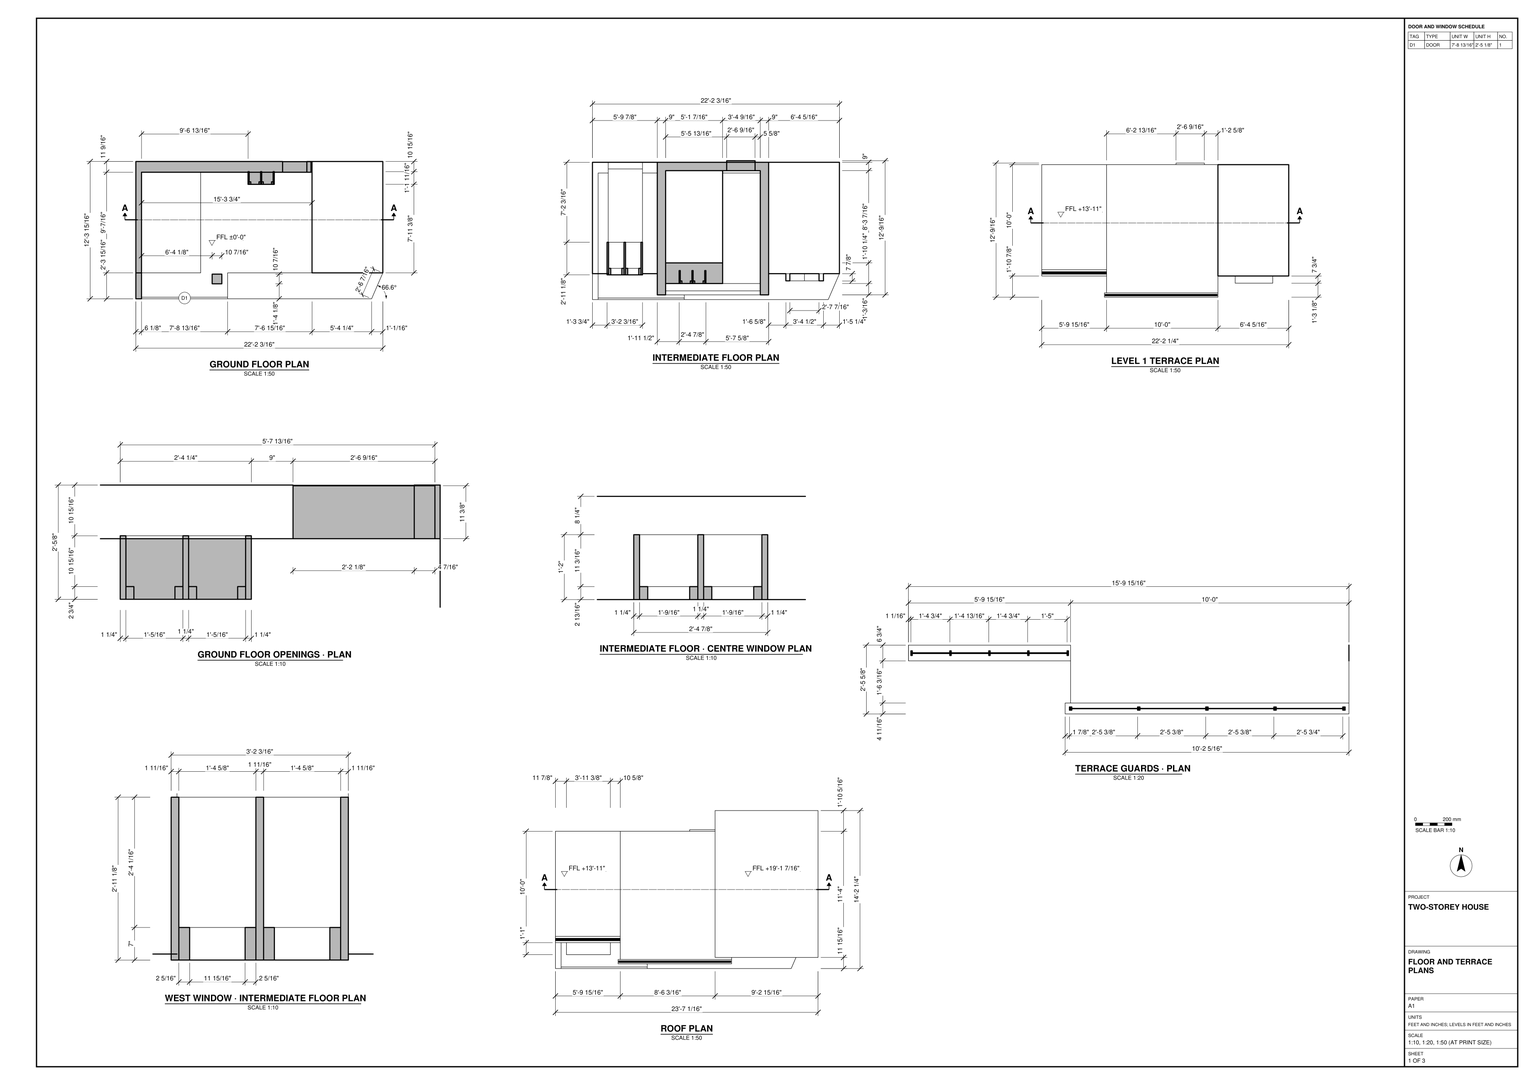
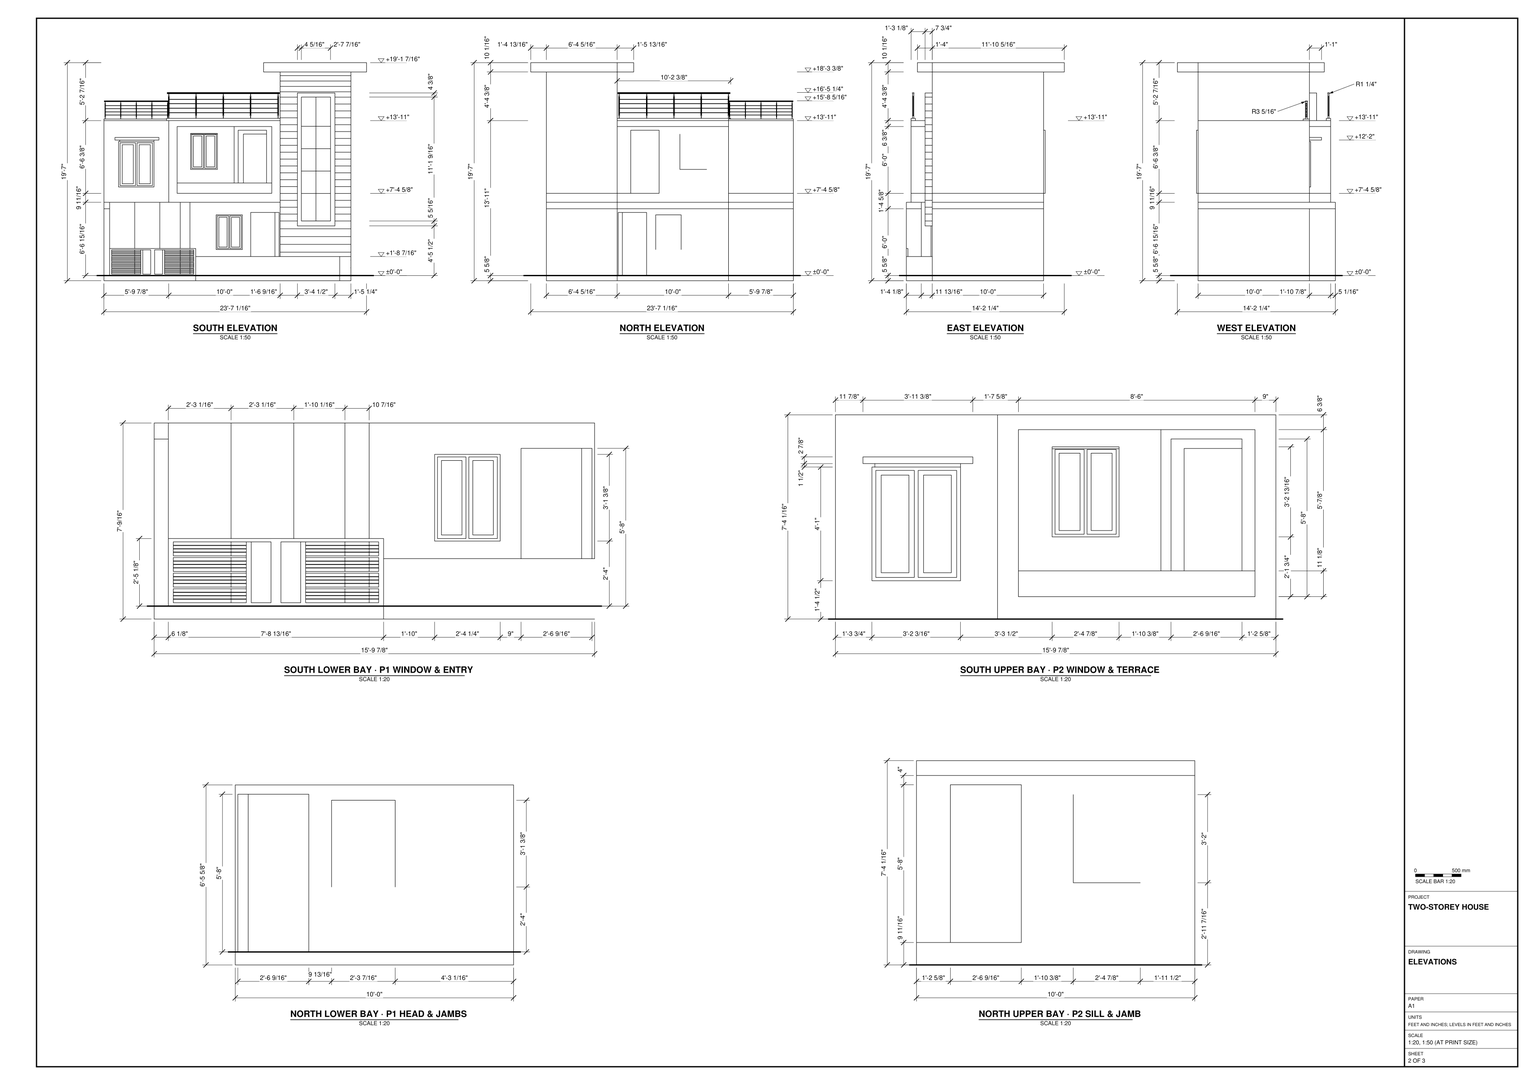
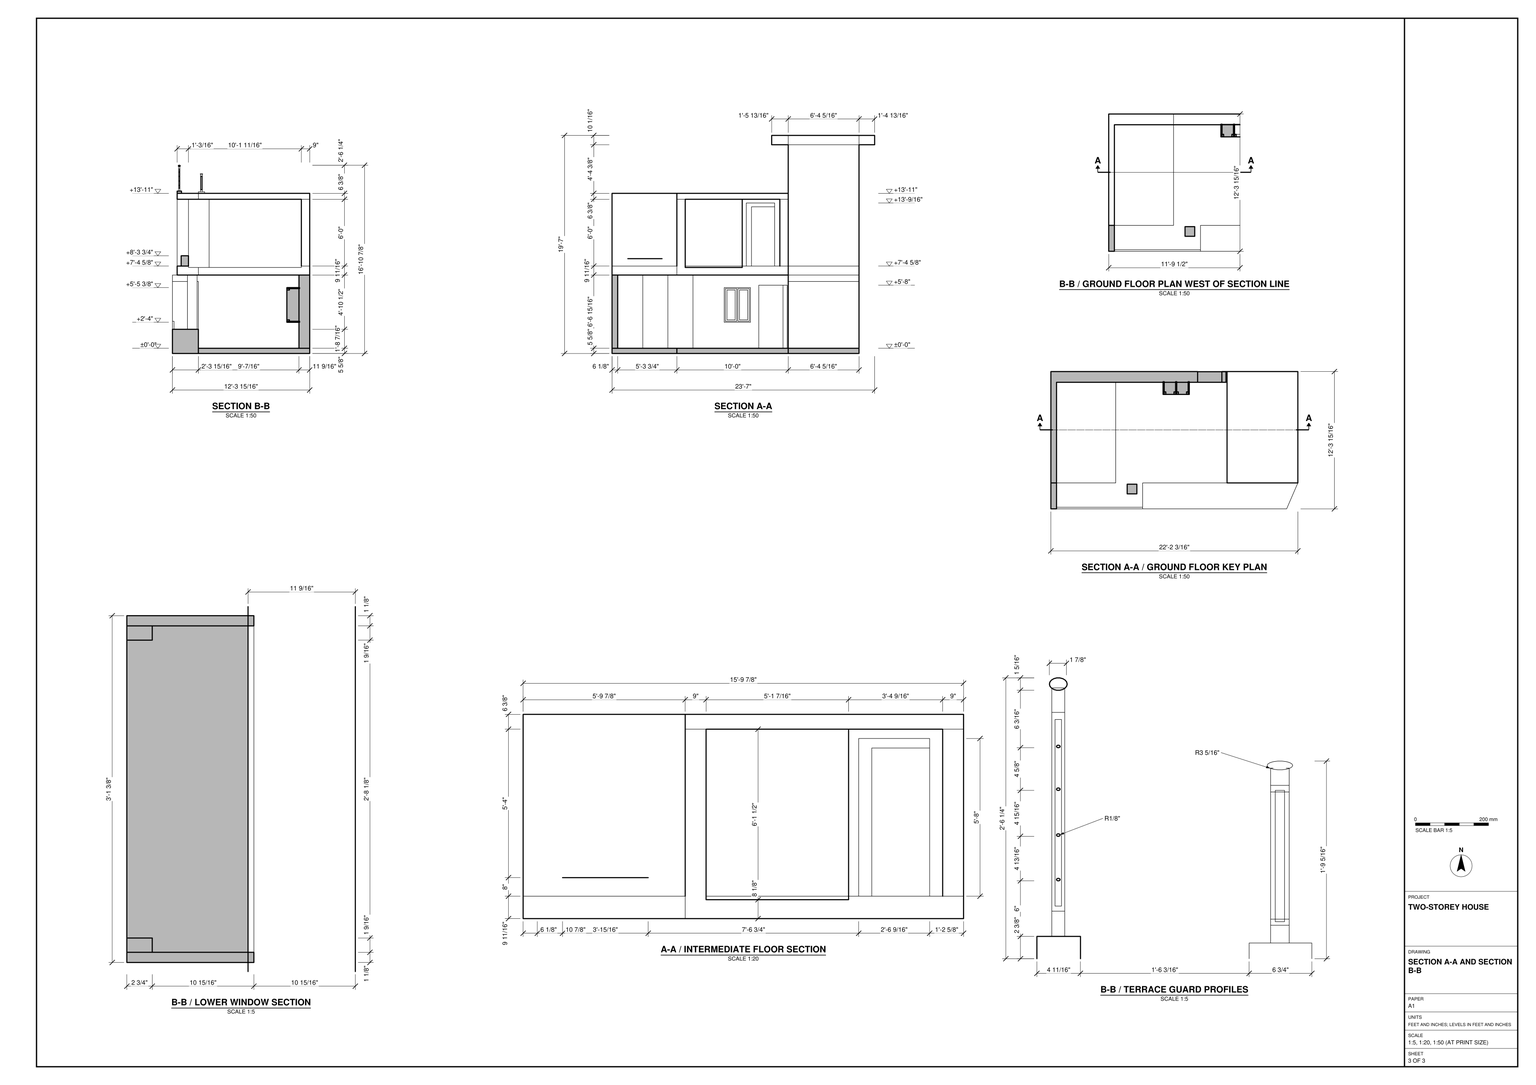
Build the two-storey house in SketchUp from task_files/diagram_01.pdf. Work in feet and inches. The overall size is 23'-7 1/16" east to west, 14'-2 1/4" north to south and 19'-7" high. Set the ground floor at ±0'-0" and the terrace at +13'-11". Use the sections to place the intermediate floor between these levels and to establish the slab thicknesses.

Follow the footprints on the floor plans, including the angled corner at the southeast of the ground floor. Give the walls their drawn thicknesses and form the door and window openings with their frames, sills and recesses. On the south elevation, model the low entry gate, the upper west window beneath its projecting head, and the recessed upper bay with a window and door. Give the taller east bay its horizontal bands, tall divided window and overhanging flat roof. Follow the terrace plan for the offset guard runs and the elevations for their different heights.

Keep the walls, slabs and roof as separate groups or components, and group each joinery or furniture piece separately where shown. Use components for repeated parts. Any decor or loose items may be suitable library components. Save one SketchUp model as output_files/two_storey_house_with_stepped_terraces_and_a_tower_bay.skp.

# SketchUp Ruby script. Lengths in inches.
U = 1.inch
M = Sketchup.active_model
def pt(a) = Geom::Point3d.new(a.map { |v| v * U })
def face(e, loops, mat)
  f = e.add_face(loops[0].map { |a| pt(a) })
  loops[1..].each { |l| e.add_face(l.map { |a| pt(a) }).erase! }
  f.material = f.back_material = mat if mat
  f
end
# faces: each face lists its corners as indices into pts; further lists are holes
def faces(e, pts, list, mat = nil) = list.each { |f| face(e, (f[0].is_a?(Array) ? f : [f]).map { |l| l.map { |i| pts[i] } }, mat) }
# xy, xz, yz: faces in a plane at the given z, y or x. An outline is a flat list of corners, or four numbers for a rectangle; further outlines are holes
def ring(l) = l.size == 4 ? [[l[0], l[1]], [l[2], l[1]], [l[2], l[3]], [l[0], l[3]]] : l.each_slice(2).to_a
def flat(e, list, mat, &to3) = list.each { |f| face(e, (f[0].is_a?(Array) ? f : [f]).map { |l| ring(l).map { |u, v| to3.(u, v) } }, mat) }
def xy(e, z, list, mat = nil) = flat(e, list, mat) { |x, y| [x, y, z] }
def xz(e, y, list, mat = nil) = flat(e, list, mat) { |x, z| [x, y, z] }
def yz(e, x, list, mat = nil) = flat(e, list, mat) { |y, z| [x, y, z] }
def lines(e, pts, list) = list.each { |a, b| e.add_line(pt(pts[a]), pt(pts[b])) }
# prism: a flat outline (further loops are holes) pulled along v
def prism(e, loops, v, mat = nil)
  f = face(e, loops, mat); d = Geom::Vector3d.new(v.map { |x| x * U })
  f.pushpull(f.normal.samedirection?(d) ? d.length : -d.length)
end
def box(e, o, s, mat = nil) = prism(e, [[o, [o[0] + s[0], o[1], o[2]], [o[0] + s[0], o[1] + s[1], o[2]], [o[0], o[1] + s[1], o[2]]]], [0, 0, s[2]], mat)
def at(x, y, z, deg = 0) = Geom::Transformation.translation(pt([x, y, z])) * Geom::Transformation.rotation(ORIGIN, Z_AXIS, deg.degrees)
def axes(o, x, y, z) = Geom::Transformation.new([*x, 0, *y, 0, *z, 0, *pt(o).to_a, 1])
def part(name) = M.definitions.add(name)
# library, detail: a bought-in or finely detailed component or shape, given as its bounding box
def library(name, o, s) = part(name).tap { |d| box(d.entities, o, s) }
def detail(e, o, s) = box(e.add_group.entities, o, s)
def put(e, d, t, mat = nil) = e.add_instance(d, t).tap { |i| i.material = mat if mat }
def group(e, t, mat = nil) = e.add_group.tap { |g| g.transformation = t; g.material = mat if mat }.entities
root = M.entities
M.materials.add("JJJ1").color = [238, 218, 183]
M.materials.add("MU TIGHI 6T67L 1").color = [235, 235, 235]
M.materials.add("T ER5Y 565N 1").color = [201, 111, 22]
M.materials.add("T R72 56 8, 7 5U1").color = [25, 25, 25]
M.materials.add("[Color I02]").color = [170, 141, 255]
M.materials["[Color I02]"].alpha = 0.92
M.materials.add("[Color J02]").color = [244, 207, 255]
M.materials.add("[Color J07]").color = [2, 0, 62]
M.materials.add("[Color M08]").color = [30, 30, 30]
M.materials.add("[Translucent Glass Blue]").color = [100, 149, 237]
M.materials["[Translucent Glass Blue]"].alpha = 0.18
M.materials.add("[Translucent Glass Gray]1").color = [132, 132, 132]
M.materials["[Translucent Glass Gray]1"].alpha = 0.25
M.materials.add("[Wood Plywood Knots]").color = [137, 122, 41]
M.materials.add("[Wood Veneer 01]").color = [120, 70, 37]
M.materials.add("wefsd tger 1").color = [92, 92, 92]
c1 = part("Group\#8")
xy(c1.entities,0,[[0,0,19.69,1.18]],"[Wood Veneer 01]")
xy(c1.entities,2.76,[[2.76,0,16.93,1.18]],"[Wood Veneer 01]")
xy(c1.entities,60.24,[[2.76,0,16.93,1.18]],"[Wood Veneer 01]")
xy(c1.entities,62.99,[[0,0,19.69,1.18]],"[Wood Veneer 01]")
xz(c1.entities,0,[[2.76,2.76,16.93,60.24]],"[Translucent Glass Gray]1")
xz(c1.entities,0,[[[0,0,19.69,62.99],[2.76,2.76,16.93,60.24]]],"[Wood Veneer 01]")
xz(c1.entities,1.18,[[[0,0,19.69,62.99],[2.76,2.76,16.93,60.24]]],"[Wood Veneer 01]")
yz(c1.entities,0,[[0,0,1.18,62.99]],"[Wood Veneer 01]")
yz(c1.entities,2.76,[[0,2.76,1.18,60.24]],"[Wood Veneer 01]")
yz(c1.entities,16.93,[[0,2.76,1.18,60.24]],"[Wood Veneer 01]")
yz(c1.entities,19.69,[[0,0,1.18,62.99]],"[Wood Veneer 01]")
c2 = part("pintu 2")
put(c2.entities,c1,at(-19.69,0,1.97))
g1 = group(c2.entities,at(-21.65,0,0))
prism(g1,[[[0,0,66.93],[0,0,0],[45.28,0,0],[45.28,0,66.93]],[[43.31,0,1.97],[23.62,0,1.97],[23.62,0,64.96],[43.31,0,64.96]],[[21.65,0,64.96],[21.65,0,1.97],[1.97,0,1.97],[1.97,0,64.96]]],[0,5.91,0],"[Wood Veneer 01]")
put(c2.entities,c1,at(1.97,0,1.97))
c3 = part("DOOR12")
g2 = group(c3.entities,at(114.73,28.14,-0.51))
g3 = group(g2,at(0,0,0))
box(g3,[0,0,0],[36,0.5,77.7])
c4 = part("Box01")
box(c4.entities,[-251.12,-5.93,-8.91],[582.61,12.27,8.91],"wefsd tger 1")
c5 = part("Box45")
box(c5.entities,[-240.91,-0.82,12.1],[2.44,1.82,74.48],"JJJ1")
c6 = part("Cylinder01")
prism(c6.entities,[[[328.21,-1.16,98.56],[328.21,-0.34,98.26],[328.21,0.53,98.26],[328.21,1.34,98.56],[328.21,2.01,99.11],[328.21,2.44,99.87],[328.21,2.59,100.72],[328.21,2.44,101.58],[328.21,2.01,102.33],[328.21,1.34,102.89],[328.21,0.53,103.18],[328.21,-0.34,103.18],[328.21,-1.16,102.89],[328.21,-1.82,102.33],[328.21,-2.25,101.58],[328.21,-2.41,100.72],[328.21,-2.25,99.87],[328.21,-1.82,99.11]]],[-576.3,0,0],"T ER5Y 565N 1")
c7 = part("Cylinder02")
prism(c7.entities,[[[-239.93,0.18,76.32],[-239.93,0.34,76.26],[-239.93,0.48,76.15],[-239.93,0.5625,75.99],[-239.93,0.59,75.82],[-239.93,0.5625,75.65],[-239.93,0.48,75.5],[-239.93,0.34,75.39],[-239.93,0.18,75.33],[-239.93,0.01,75.33],[-239.93,-0.16,75.39],[-239.93,-0.29,75.5],[-239.93,-0.375,75.65],[-239.93,-0.41,75.82],[-239.93,-0.375,75.99],[-239.93,-0.29,76.15],[-239.93,-0.16,76.26],[-239.93,0.01,76.32]]],[560.05,0,0],"T R72 56 8, 7 5U1")
c8 = part("Rectangle1")
prism(c8.entities,[[[-237.41,1.91,10.08],[-239.22,1.91,10.08],[-239.22,1.91,0.02],[-240.41,1.91,0.02],[-240.41,1.91,10.08],[-242.22,1.91,10.08],[-242.22,1.91,89.41],[-240.41,1.91,89.41],[-240.41,1.91,99.1875],[-239.22,1.91,99.1875],[-239.22,1.91,89.41],[-237.41,1.91,89.41]],[[-240.4375,1.91,85.68],[-240.4375,1.91,13.53],[-239.08,1.91,13.53],[-239.08,1.91,85.68]]],[0,-3.64,0],"MU TIGHI 6T67L 1")
c9 = part("skp243")
put(c9.entities,c4,at(0,0,0))
put(c9.entities,c5,at(0,0,0))
put(c9.entities,c6,at(0,0,0))
put(c9.entities,c7,at(0,0,0))
put(c9.entities,c8,at(0,0,0))
put(c9.entities,c7,at(0,0,-17.07))
put(c9.entities,c7,at(0,0,-35.38))
put(c9.entities,c7,at(0,0,-53.15))
put(c9.entities,c5,at(139.83,0,0))
put(c9.entities,c8,at(139.83,0,0))
put(c9.entities,c8,at(279.78,0,0))
put(c9.entities,c5,at(279.78,0,0))
put(c9.entities,c5,at(419.57,0,0))
put(c9.entities,c8,at(419.57,0,0))
put(c9.entities,c8,at(561.11,0,0))
put(c9.entities,c5,at(561.11,0,0))
c10 = part("Railing1")
put(c10.entities,c9,at(251.12,5.93,8.91))
c11 = part("1")
xy(c11.entities,0,[[0,0,58.27,0.39]])
xy(c11.entities,0.39,[[0,0,58.27,0.39]])
xy(c11.entities,3.9375,[[0,0,58.27,0.39]])
xy(c11.entities,4.33,[[0,0,58.27,0.39]])
xy(c11.entities,7.875,[[0,0,58.27,0.39]])
xy(c11.entities,8.27,[[0,0,58.27,0.39]])
xz(c11.entities,0,[[0,0,58.27,0.39],[0,3.9375,58.27,4.33],[0,7.875,58.27,8.27]])
xz(c11.entities,0.39,[[0,0,58.27,0.39],[0,3.9375,58.27,4.33],[0,7.875,58.27,8.27]])
c12 = part("gate")
xy(c12.entities,0,[[0,0,171.26,1.97]])
xy(c12.entities,3.9375,[[3.9375,0,62.01,1.97],[65.94,0,81.69,0.39],[89.57,0,105.31,0.39],[109.25,0,167.32,1.97],[65.94,0.98,81.69,1.97],
  [89.57,0.98,105.31,1.97]])
xy(c12.entities,20.18,[[3.9375,0,62.01,1.97],[109.25,0,167.32,1.97]])
xy(c12.entities,22.15,[[3.9375,0,62.01,1.97],[109.25,0,167.32,1.97]])
xy(c12.entities,38.39,[[3.9375,0,62.01,1.97],[109.25,0,167.32,1.97]])
xy(c12.entities,40.35,[[3.9375,0,62.01,1.97],[109.25,0,167.32,1.97]])
xy(c12.entities,56.59,[[3.9375,0,62.01,1.97],[109.25,0,167.32,1.97]])
xy(c12.entities,58.5625,[[3.9375,0,62.01,1.97],[109.25,0,167.32,1.97]])
xy(c12.entities,62.6,[[3.9375,0.59,62.2,0.98]])
xy(c12.entities,62.99,[[3.9375,0.59,62.2,0.98]])
xy(c12.entities,66.54,[[3.9375,0.59,62.2,0.98]])
xy(c12.entities,66.93,[[3.9375,0.59,62.2,0.98]])
xy(c12.entities,70.47,[[3.9375,0.59,62.2,0.98]])
xy(c12.entities,70.87,[[3.9375,0.59,62.2,0.98]])
xy(c12.entities,74.8,[[3.9375,0,62.01,1.97],[65.94,0,81.69,0.39],[89.57,0,105.31,0.39],[109.25,0,167.32,1.97],[65.94,0.98,81.69,1.97],
  [89.57,0.98,105.31,1.97]])
xy(c12.entities,78.74,[[0,0,171.26,1.97]])
xz(c12.entities,0,[[[0,0,85.63,78.74],[65.94,3.9375,81.69,74.8],[3.9375,22.15,62.01,38.39],[3.9375,3.9375,62.01,20.18],[3.9375,58.5625,62.01,74.8],[3.9375,40.35,62.01,56.59]],[[85.63,0,171.26,78.74],[89.57,3.9375,105.31,74.8],[109.25,22.15,167.32,38.39],[109.25,40.35,167.32,56.59],[109.25,58.5625,167.32,74.8],[109.25,3.9375,167.32,20.18]]],"[Color M08]")
xz(c12.entities,0.39,[[65.94,3.9375,81.69,74.8],[89.57,3.9375,105.31,74.8]],"[Wood Plywood Knots]")
xz(c12.entities,0.59,[[3.9375,62.6,62.2,62.99],[3.9375,66.54,62.2,66.93],[3.9375,70.47,62.2,70.87]])
xz(c12.entities,0.98,[[65.94,3.9375,81.69,74.8],[89.57,3.9375,105.31,74.8],[3.9375,62.6,62.2,62.99],[3.9375,66.54,62.2,66.93],[3.9375,70.47,62.2,70.87]])
xz(c12.entities,1.97,[[[0,0,171.26,78.74],[65.94,3.9375,81.69,74.8],[89.57,3.9375,105.31,74.8],[109.25,40.35,167.32,56.59],[109.25,22.15,167.32,38.39],[3.9375,3.9375,62.01,20.18],[3.9375,22.15,62.01,38.39],[109.25,58.5625,167.32,74.8],[3.9375,40.35,62.01,56.59],[3.9375,58.5625,62.01,74.8],[109.25,3.9375,167.32,20.18]]])
yz(c12.entities,0,[[0,0,1.97,78.74]])
yz(c12.entities,3.9375,[[0,3.9375,0.98,20.18],[0.98,3.9375,1.97,20.18],[0,22.15,0.98,38.39],[0.98,22.15,1.97,38.39],[0,40.35,0.98,56.59],
  [0.98,40.35,1.97,56.59],[0,58.5625,0.98,58.5625,0.98,62.6,0.59,62.6,0.59,62.99,0.98,62.99,0.98,66.54,0.59,66.54,0.59,66.93,0.98,66.93,0.98,70.47,0.59,70.47,0.59,70.87,0.98,70.87,0.98,74.8,0,74.8],[0.98,58.5625,1.97,74.8]])
yz(c12.entities,62.01,[[0,3.9375,1.97,20.18],[0,20.18,1.97,22.15],[0,22.15,1.97,38.39],[0,40.35,1.97,56.59],[0,58.5625,1.97,74.8]])
yz(c12.entities,62.2,[[0.59,62.6,0.98,62.99],[0.59,66.54,0.98,66.93],[0.59,70.47,0.98,70.87]])
yz(c12.entities,65.94,[[0,3.9375,0.39,74.8],[0.98,3.9375,1.97,74.8]])
yz(c12.entities,81.69,[[0,3.9375,0.39,74.8],[0.98,3.9375,1.97,74.8]])
yz(c12.entities,89.57,[[0,3.9375,0.39,74.8],[0.98,3.9375,1.97,74.8]])
yz(c12.entities,105.31,[[0,3.9375,0.39,74.8],[0.98,3.9375,1.97,74.8]])
yz(c12.entities,109.25,[[0,3.9375,1.97,20.18],[0,20.18,1.97,22.15],[0,22.15,1.97,38.39],[0,38.39,1.97,40.35],[0,40.35,1.97,56.59],
  [0,56.59,1.97,58.5625],[0,58.5625,1.97,74.8]])
yz(c12.entities,167.32,[[0,3.9375,1.97,20.18],[0,22.15,1.97,38.39],[0,40.35,1.97,56.59],[0,58.5625,1.97,74.8]])
yz(c12.entities,171.26,[[0,0,1.97,78.74]])
p = [[65.94,0.39,74.8],[65.94,0.98,74.8],[105.31,0.39,74.8],[105.31,0.98,74.8],[62.01,1.97,74.8],[65.94,1.97,74.8],
  [105.31,1.97,74.8],[109.25,1.97,74.8],[62.01,1.97,38.39],[62.01,1.97,40.35],[62.01,1.97,56.59],[62.01,1.97,58.5625],
  [3.9375,0.98,22.15],[3.9375,0.98,20.18],[3.9375,0.98,40.35],[3.9375,0.98,38.39],[3.9375,0.98,58.5625],[3.9375,0.98,56.59]]
lines(c12.entities,p,[[0,1],[2,3],[4,5],[6,7],[8,9],[10,11],[12,13],[14,15],[16,17]])
put(c12.entities,c11,at(3.9375,0.59,44.39))
put(c12.entities,c11,at(3.9375,0.59,7.97))
put(c12.entities,c11,at(109.25,0.62,62.6))
put(c12.entities,c11,at(109.25,0.68,44.33))
put(c12.entities,c11,at(109.25,0.68,26.22))
put(c12.entities,c11,at(109.25,0.68,8.11))
put(c12.entities,c11,at(3.9375,0.59,26.18))
xy(root,-5.6,[[0.04,0,69.91,27.9375],[69.91,0,98.95,27.9375],[98.95,0,98.95,27.9375,266.23,27.9375,254.14,0],[0.04,27.9375,69.91,147.9375],[69.91,27.9375,189.91,147.9375],
  [189.91,27.9375,266.23,147.9375]])
xy(root,-2.25,[[82.28,16.13,92.72,26.57]])
xy(root,0,[[0.04,0,6.15,27.9375],[6.15,0,98.95,0,98.95,27.9375,189.91,27.9375,189.91,136.375,184.33,136.375,184.33,147.9375,158.2,147.9375,158.2,136.375,69.91,136.375,69.91,27.9375,6.15,27.9375],[0.04,27.9375,0.04,147.9375,69.91,147.9375,69.91,136.375,6.15,136.375,6.15,27.9375],[6.15,27.9375,69.91,136.375],[189.91,27.9375,266.23,147.9375],
  [69.91,136.375,158.2,147.9375],[184.33,136.375,189.91,147.9375]])
xy(root,20.47,[[98.95,0,254.14,0,266.23,27.9375,98.95,27.9375]])
xy(root,53.47,[[208.5,20.1875,249,27.9375]])
xy(root,58.83,[[212.8,20.1875,228.52,27.9375],[228.52,20.1875,244.24,27.9375]])
xy(root,67.99,[[158.2,136.375,184.33,147.9375]])
xy(root,72,[[0.04,0,6.15,27.9375]])
xy(root,78.9375,[[0.04,0,6.15,27.9375],[[69.91,5.0625,69.91,27.9375,6.15,27.9375,6.15,136.375,189.91,136.375,189.91,5.0625],[82.28,16.13,92.72,26.57]],[82.28,16.13,92.72,26.57],[0.04,27.9375,0.04,147.9375,69.91,147.9375,69.91,136.375,6.15,136.375,6.15,27.9375],[69.91,136.375,189.91,147.9375]])
xy(root,87.09,[[78.91,17.28,140.35,39.53],[78.91,39.53,140.35,138.9375]])
xy(root,88.59,[[78.91,5.0625,180.91,9.39],[78.91,9.39,180.91,17.28]])
xy(root,96.59,[[17.03,27.9375,53.96,140.77]])
xy(root,99.72,[[78.91,9.39,180.91,17.28]])
xy(root,145.97,[[11.89,14.9375,17.03,27.9375],[17.03,14.9375,53.96,27.9375],[53.96,14.9375,59.28,27.9375]])
xy(root,148.84,[[11.89,14.9375,59.28,27.9375]])
xy(root,160.59,[[78.91,5.0625,78.91,17.28,140.35,17.28,140.35,138.9375,180.91,138.9375,180.91,5.0625],[78.91,17.28,140.35,39.53],[78.91,39.53,140.35,138.9375]])
xy(root,166.98,[[69.91,5.0625,189.91,147.9375],[0.04,27.9375,69.91,147.9375]])
xy(root,192.33,[[212.8,20.1875,228.52,27.9375],[228.52,20.1875,244.24,27.9375]])
xy(root,196.72,[[208.5,20.1875,249,27.9375]])
xy(root,219.36,[[172.1,11.9375,283.07,27.9375],[172.1,27.9375,189.91,170.25],[266.23,27.9375,266.23,147.9375,189.91,147.9375,189.91,170.25,283.07,170.25,283.07,27.9375]])
xy(root,229.42,[[172.1,11.9375,283.07,170.25]])
xz(root,0,[[0.04,-5.6,98.95,0],[98.95,-5.6,254.14,20.47],[0.04,0,6.15,72],[0.04,72,6.15,78.9375]])
xz(root,5.0625,[[[69.91,78.9375,189.91,166.98],[78.91,88.59,180.91,160.59]]],"[Color J07]")
xz(root,9.39,[[78.91,88.59,180.91,99.72]],"[Color I02]")
xz(root,11.9375,[[172.1,219.36,283.07,229.42]])
xz(root,14.9375,[[11.89,145.97,59.28,148.84]])
xz(root,16.13,[[82.28,-2.25,92.72,78.9375]])
xz(root,17.28,[[78.91,87.09,140.35,88.59],[78.91,88.59,140.35,99.72],[140.35,88.59,180.91,99.72],[[78.91,99.72,140.35,160.59],[93.44,114.36,122.32,152.36]]])
xz(root,20.1875,[[[208.5,53.47,249,196.72],[212.8,58.83,244.24,192.33]]])
xz(root,26.57,[[82.28,-2.25,92.72,78.9375]])
xz(root,27.9375,[[0.04,-5.6,69.91,0],[98.95,-5.6,189.91,0],[189.91,-5.6,266.23,0],[0.04,0,6.15,72],[98.95,0,189.91,20.47],
  [189.91,0,266.23,8.4],[189.91,8.4,266.23,16.79],[189.91,16.79,266.23,20.47],[189.91,20.47,266.23,25.19],[189.91,25.19,266.23,33.59],
  [189.91,33.59,266.23,41.99],[189.91,41.99,266.23,50.38],[189.91,50.38,266.23,50.38,266.23,58.78,249,58.78,249,53.47,208.5,53.47,208.5,58.78,189.91,58.78],[189.91,58.78,208.5,66.19],[249,58.78,266.23,66.19],
  [189.91,66.19,208.5,73.61],[249,66.19,266.23,73.61],[189.91,73.61,208.5,81.02],[249,73.61,266.23,81.02],[189.91,81.02,208.5,88.4375],
  [249,81.02,266.23,88.4375],[189.91,88.4375,208.5,95.85],[249,88.4375,266.23,95.85],[189.91,95.85,208.5,103.26],[249,95.85,266.23,103.26],
  [189.91,103.26,208.5,110.68],[249,103.26,266.23,110.68],[189.91,110.68,208.5,118.09],[249,110.68,266.23,118.09],[189.91,118.09,208.5,125.51],
  [249,118.09,266.23,125.51],[189.91,125.51,208.5,132.92],[249,125.51,266.23,132.92],[189.91,132.92,208.5,140.34],[249,132.92,266.23,140.34],
  [189.91,140.34,208.5,147.75],[249,140.34,266.23,147.75],[11.89,145.97,59.28,148.84],[189.91,147.75,208.5,155.16],[249,147.75,266.23,155.16],
  [189.91,155.16,208.5,162.58],[249,155.16,266.23,162.58],[189.91,162.58,208.5,169.99],[249,162.58,266.23,169.99],[189.91,169.99,208.5,177.41],
  [249,169.99,266.23,177.41],[189.91,177.41,208.5,184.82],[249,177.41,266.23,184.82],[189.91,184.82,208.5,192.23],[249,184.82,266.23,192.23],
  [189.91,192.23,208.5,192.23,208.5,196.72,249,196.72,249,192.23,266.23,192.23,266.23,198.03,189.91,198.03],[189.91,198.03,266.23,203.83],[189.91,203.83,266.23,209.625],[189.91,209.625,266.23,215.42],[189.91,215.42,266.23,219.36]])
xz(root,27.9375,[[[0.04,78.9375,69.91,166.98],[17.03,96.59,17.03,145.97,11.89,145.97,11.89,148.84,59.28,148.84,59.28,145.97,53.96,145.97,53.96,96.59]]],"[Color J02]")
xz(root,27.9375,[[212.8,58.83,228.52,88.44],[228.52,58.83,244.24,88.44],[212.8,88.44,228.52,112.56],[228.52,88.44,244.24,112.56],[212.8,112.56,228.52,136.69],
  [228.52,112.56,244.24,136.69],[212.8,136.69,228.52,160.81],[228.52,136.69,244.24,160.81],[212.8,160.81,228.52,192.33],[228.52,160.81,244.24,192.33]],"[Translucent Glass Blue]")
xz(root,39.53,[[78.91,87.09,140.35,160.59]])
xz(root,136.375,[[6.15,0,33.19,78.9375],[33.19,0,60.23,78.9375],[60.23,0,87.27,78.9375],[87.27,0,158.2,0,158.2,67.99,184.33,67.99,184.33,0,189.91,0,189.91,78.9375,87.27,78.9375]])
xz(root,138.9375,[[78.91,87.09,140.35,88.59],[78.91,88.59,140.35,160.59],[140.35,88.59,150.35,88.59,150.35,152.47,175.3,152.47,175.3,88.59,180.91,88.59,180.91,160.59,140.35,160.59]])
xz(root,147.9375,[[0.04,-5.6,69.91,0],[69.91,-5.6,189.91,0],[189.91,-5.6,266.23,0],[0.04,0,69.91,72],[69.91,0,69.91,72,189.91,72,189.91,0,184.33,0,184.33,67.99,158.2,67.99,158.2,0],
  [189.91,0,266.23,72],[0.04,72,69.91,78.9375],[69.91,72,189.91,78.9375],[189.91,72,266.23,78.9375],[0.04,78.9375,69.91,88.59],
  [69.91,78.9375,189.91,160.59],[189.91,78.9375,266.23,88.59],[0.04,88.59,69.91,166.98],[189.91,88.59,266.23,219.36],[69.91,160.59,189.91,166.98]])
xz(root,170.25,[[172.1,219.36,189.91,229.42],[189.91,219.36,283.07,229.42]])
yz(root,0.04,[[0,-5.6,27.9375,0],[27.9375,-5.6,147.9375,0],[0,0,27.9375,72],[27.9375,0,147.9375,72],[0,72,147.9375,78.9375],
  [27.9375,78.9375,147.9375,88.59],[27.9375,88.59,147.9375,166.98]])
yz(root,6.15,[[0,0,27.9375,72],[27.9375,0,136.375,0,136.375,78.9375,0,78.9375,0,72,27.9375,72]])
yz(root,11.89,[[14.9375,145.97,27.9375,148.84]])
yz(root,59.28,[[14.9375,145.97,27.9375,148.84]])
yz(root,69.91,[[27.9375,-5.6,147.9375,0],[5.0625,78.9375,27.9375,88.59],[5.0625,88.59,27.9375,160.59],[27.9375,88.59,147.9375,160.59],[5.0625,160.59,27.9375,166.98],
  [27.9375,160.59,147.9375,166.98]])
yz(root,78.91,[[17.28,87.09,39.53,88.59],[39.53,87.09,138.9375,88.59],[5.0625,88.59,9.39,88.59,9.39,99.72,17.28,99.72,17.28,160.59,5.0625,160.59],[9.39,88.59,17.28,99.72],[17.28,88.59,39.53,160.59],
  [39.53,88.59,138.9375,160.59]])
yz(root,82.28,[[16.13,-2.25,26.57,78.9375]])
yz(root,92.72,[[16.13,-2.25,26.57,78.9375]])
yz(root,98.95,[[0,-5.6,27.9375,0],[0,0,27.9375,20.47]])
yz(root,140.35,[[17.28,87.09,39.53,160.59],[39.53,87.09,138.9375,160.59]])
yz(root,158.2,[[136.375,0,147.9375,67.99]])
yz(root,172.1,[[11.9375,219.36,27.9375,229.42],[27.9375,219.36,147.9375,229.42],[147.9375,219.36,170.25,229.42]])
yz(root,180.91,[[5.0625,88.59,5.0625,160.59,138.9375,160.59,138.9375,88.59,17.28,88.59,17.28,99.72,9.39,99.72,9.39,88.59],[9.39,88.59,17.28,99.72]])
yz(root,184.33,[[136.375,0,147.9375,67.99]])
yz(root,189.91,[[27.9375,-5.6,147.9375,0],[27.9375,0,136.375,78.9375],[136.375,0,147.9375,72],[136.375,72,147.9375,78.9375],[5.0625,78.9375,27.9375,88.59],
  [27.9375,78.9375,147.9375,88.59],[5.0625,88.59,27.9375,160.59],[27.9375,88.59,147.9375,166.98],[5.0625,160.59,27.9375,166.98],[27.9375,166.98,147.9375,219.36]])
yz(root,208.5,[[20.1875,53.47,27.9375,66.19],[20.1875,66.19,27.9375,196.72]])
yz(root,212.8,[[20.1875,58.83,27.9375,88.44],[20.1875,88.44,27.9375,112.56],[20.1875,112.56,27.9375,136.69],[20.1875,136.69,27.9375,160.81],[20.1875,160.81,27.9375,192.33]])
yz(root,244.24,[[20.1875,58.83,27.9375,88.44],[20.1875,88.44,27.9375,112.56],[20.1875,112.56,27.9375,136.69],[20.1875,136.69,27.9375,160.81],[20.1875,160.81,27.9375,192.33]])
yz(root,249,[[20.1875,53.47,27.9375,58.78],[20.1875,58.78,27.9375,66.19],[20.1875,66.19,27.9375,73.61],[20.1875,73.61,27.9375,81.02],[20.1875,81.02,27.9375,88.4375],
  [20.1875,88.4375,27.9375,95.85],[20.1875,95.85,27.9375,103.26],[20.1875,103.26,27.9375,110.68],[20.1875,110.68,27.9375,118.09],[20.1875,118.09,27.9375,125.51],
  [20.1875,125.51,27.9375,132.92],[20.1875,132.92,27.9375,140.34],[20.1875,140.34,27.9375,147.75],[20.1875,147.75,27.9375,155.16],[20.1875,155.16,27.9375,162.58],
  [20.1875,162.58,27.9375,169.99],[20.1875,169.99,27.9375,177.41],[20.1875,177.41,27.9375,184.82],[20.1875,184.82,27.9375,192.23],[20.1875,192.23,27.9375,196.72]])
yz(root,266.23,[[27.9375,-5.6,147.9375,0],[27.9375,0,147.9375,72],[27.9375,72,147.9375,78.9375],[27.9375,78.9375,147.9375,88.59],[27.9375,88.59,147.9375,219.36]])
yz(root,283.07,[[11.9375,219.36,27.9375,229.42],[27.9375,219.36,170.25,229.42]])
p = [[254.14,0,-5.6],[266.23,27.9375,-5.6],[266.23,27.9375,0],[266.23,27.9375,8.4],[266.23,27.9375,16.79],[266.23,27.9375,20.47],
  [254.14,0,20.47],[189.91,147.9375,88.59],[175.3,147.9375,88.59],[69.91,147.9375,72],[69.91,136.375,72],[120.95,136.375,65.4],
  [148.39,136.375,65.4],[189.91,27.9375,229.42],[189.91,27.9375,219.36],[189.91,147.9375,229.42],[189.91,147.9375,219.36],[266.23,27.9375,229.42],
  [266.23,27.9375,219.36],[266.23,147.9375,219.36],[266.23,147.9375,229.42],[212.8,27.9375,58.78],[244.24,27.9375,58.78],[175.3,138.9375,88.59],
  [150.35,138.9375,88.59],[150.35,147.9375,88.59],[120.95,1244.4375,65.4],[148.39,1244.4375,65.4],[148.39,136.375,38.71],[148.39,136.375,28.02],
  [120.95,136.375,28.02],[148.39,1244.4375,28.02],[120.95,1244.4375,28.02],[53.96,27.9375,145.97],[53.96,147.9375,145.97],[17.03,27.9375,145.97],
  [17.03,147.9375,145.97],[53.96,140.77,96.59],[53.96,147.9375,96.59],[17.03,140.77,96.59],[17.03,147.9375,96.59],[122.32,623.15,152.36],
  [122.32,623.15,114.36],[93.44,623.15,114.36]]
faces(root,p,[[0,1,2,3,4,5,6]])
lines(root,p,[[7,8],[9,10],[11,12],[13,14],[15,16],[17,18],[19,20],[21,22],[23,8],[24,25],[26,27],[28,29],
  [30,11],[27,31],[32,26],[33,34],[35,36],[37,38],[39,40],[41,42],[42,43]])
put(root,c2,axes([107.25,17.28,114.36],[0.63776,0,0],[0,2.3688,0],[0,0,0.58]))
put(root,c2,axes([34.04,26.64,95.45],[0.84357,0,0],[0,5.94285,0],[0,0,0.73225]))
put(root,c2,axes([134.47,123.3125,28.02],[0.62425,0,0],[0,2.3186,0],[0,0,0.55843]))
put(root,c3,axes([60.73,-505.35,0.45],[0.84962,0,0],[0,22.8063,0],[0,0,0.87508]))
put(root,c3,axes([47.24,-463.78,89.04],[0.84962,0,0],[0,21.42,0],[0,0,0.87508]))
put(root,c10,axes([67.56,5.0625,166.98],[0.21,0,0],[0,0.3828,0],[0,0,0.27]))
put(root,c10,axes([0,27.9375,166.98],[0.12,0,0],[0,0.5508,0],[0,0,0.19]))
put(root,c12,axes([6.15,1.6875,0],[0.54186,0,0],[0,-0.85639,0],[0,0,0.37]))
